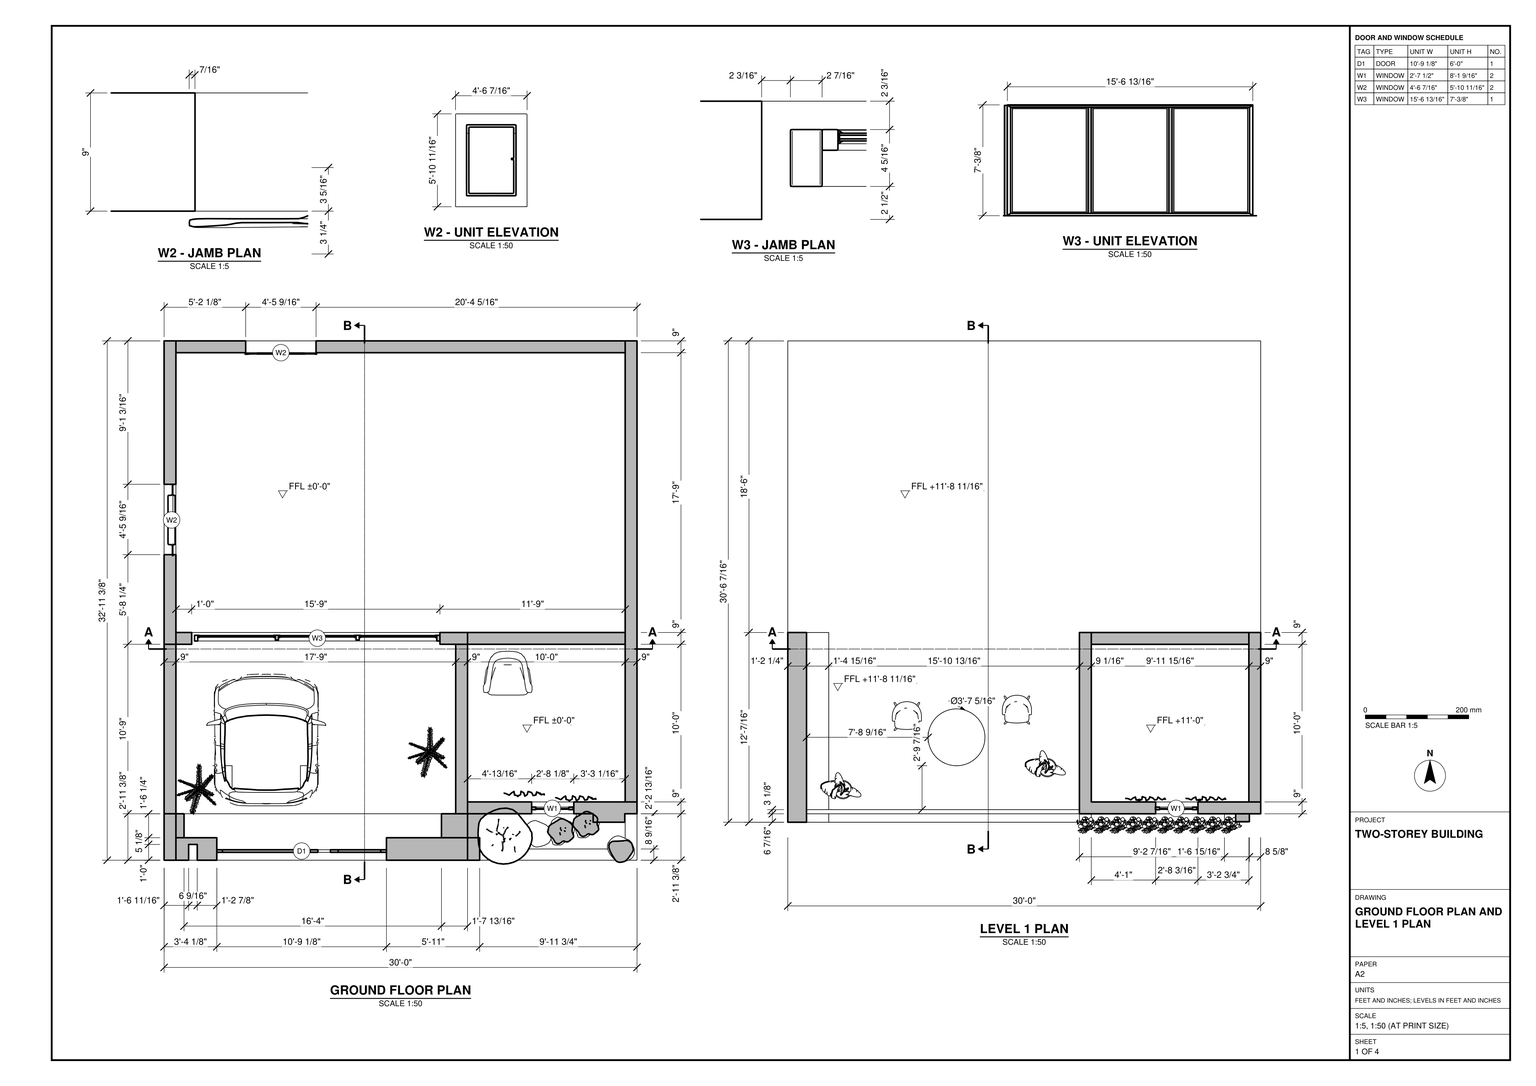
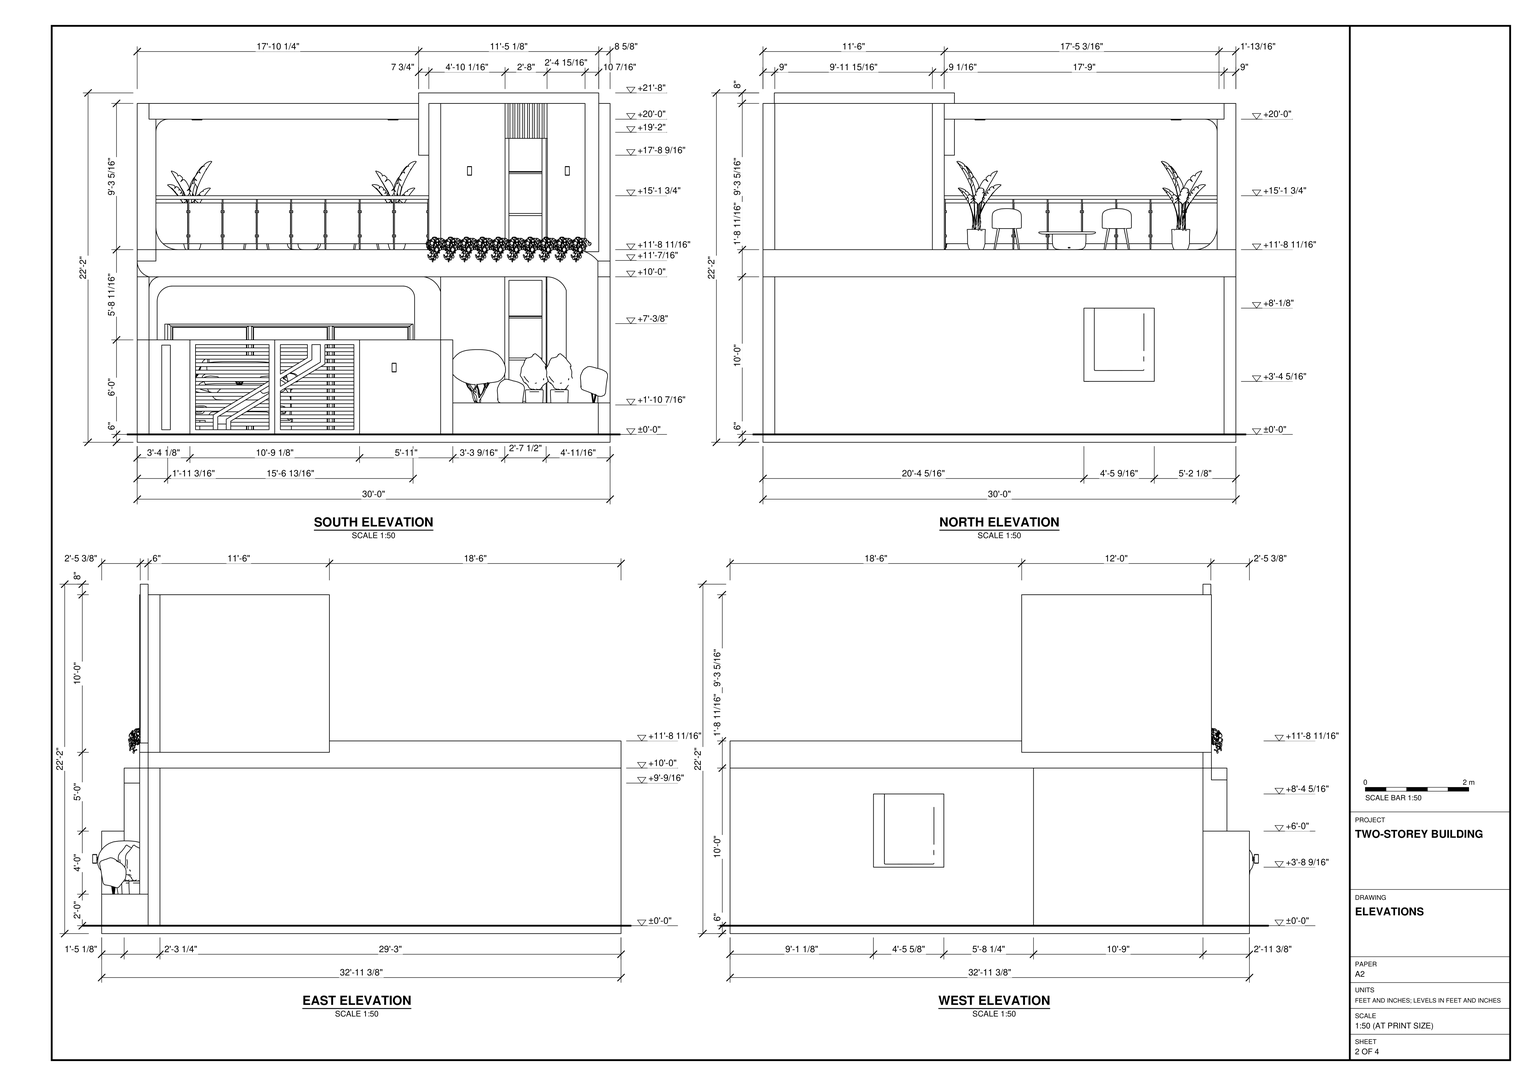
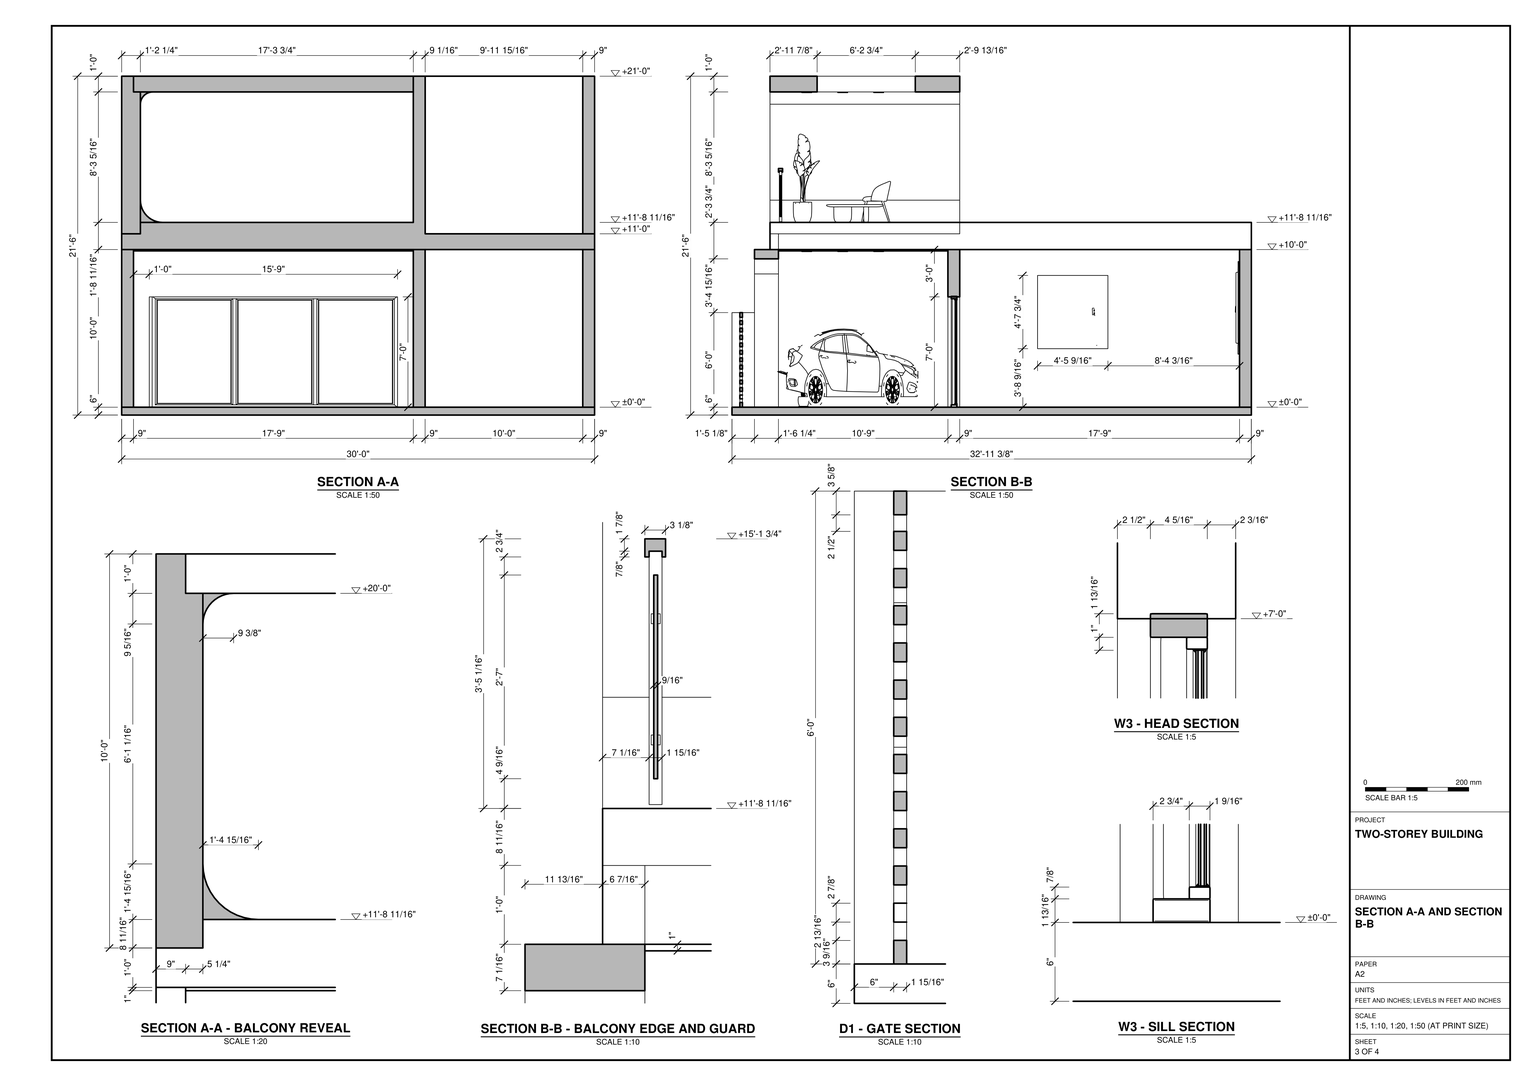
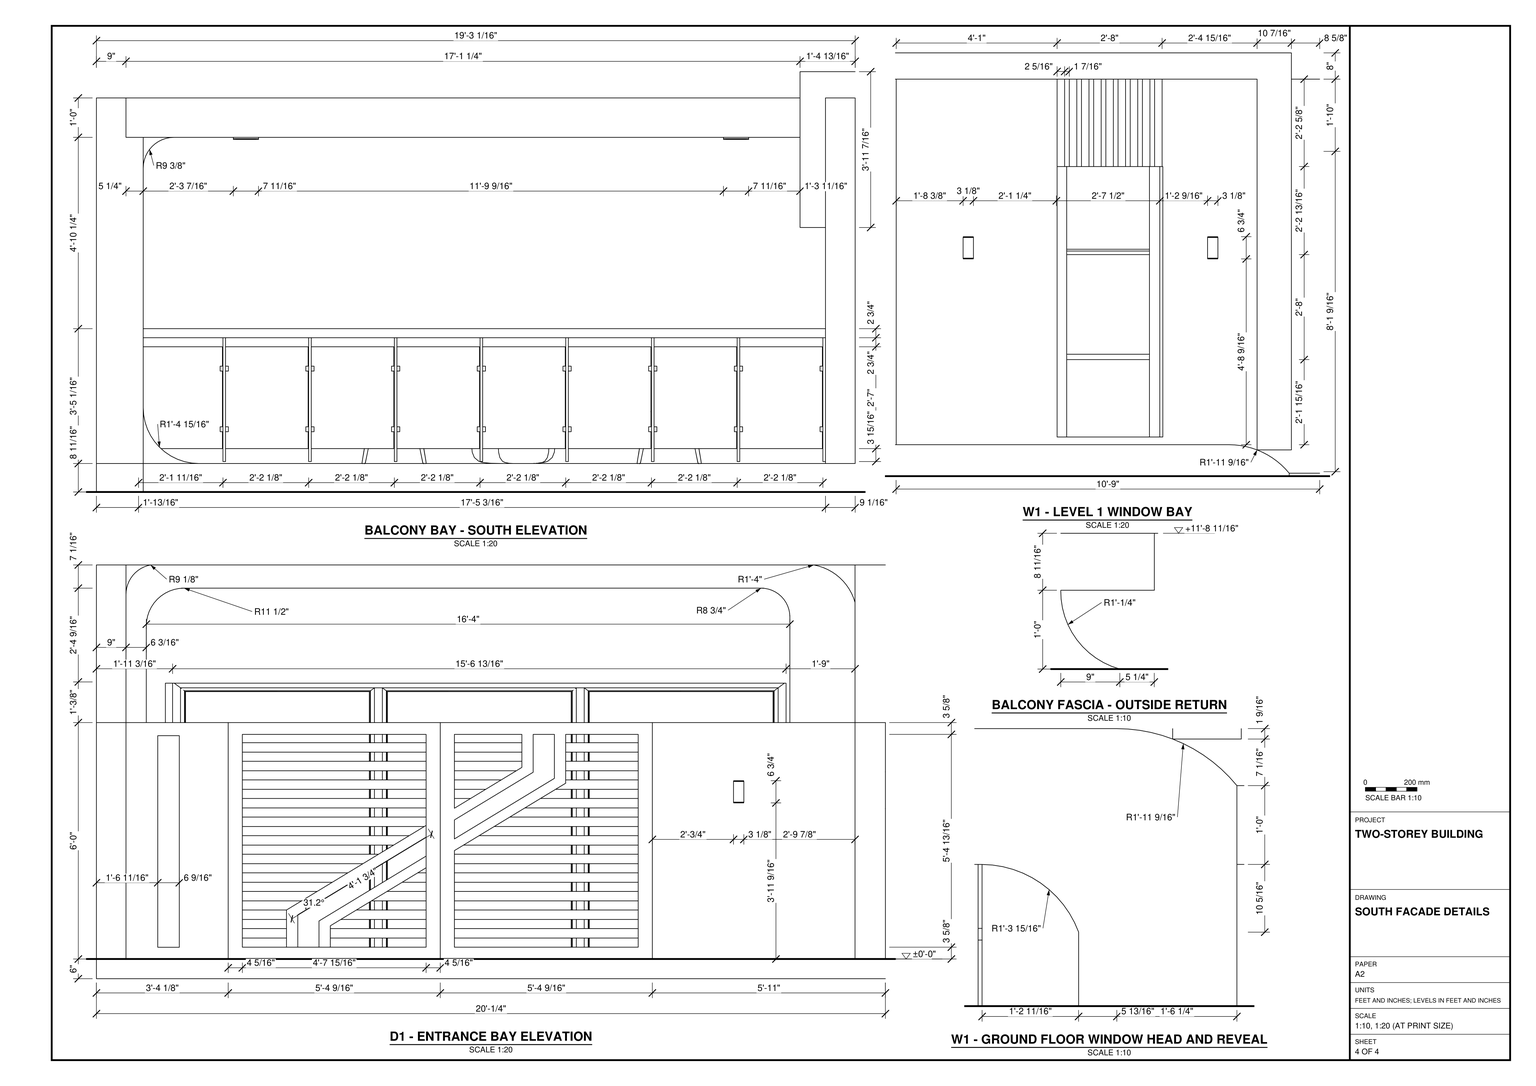
Build the two-storey building in SketchUp from task_files/diagram_01.pdf. Work in feet and inches. The overall model is 30'-0" wide, 33'-6 1/4" deep and 22'-2" high. Set the ground floor at ±0'-0" and the upper level at +11'-8 11/16".

Use the south elevation as the front. Lay out the large rear room, the covered parking bay at the front left and the smaller room at the front right. Model the walls at their drawn thicknesses, including the 9" walls shown in plan. Fit the slatted gate between the front wall piers and place the wide, three-panel window in the wall behind the parking bay. Use the plans and window schedule to locate and size the other window units.

Form the ground slab, upper slab and flat roof to match the sections. Keep the upper enclosure and covered balcony toward the front, leaving the roof surface visible behind them. Model the curved balcony reveals, stepped slab edge and glazed guard with its posts and top rail. Place the chairs and round table on the balcony, the car behind the gate and the planting as shown. Decor and loose items may be any suitable library component, for example from 3D Warehouse.

Keep the shell elements and each furniture or joinery piece in separate groups or components, and use components for repeated parts. Save one SketchUp model as output_files/two_storey_building_with_a_gated_carport_and_balcony.skp.

# SketchUp Ruby script. Lengths in inches.
U = 1.inch
M = Sketchup.active_model
def pt(a) = Geom::Point3d.new(a.map { |v| v * U })
def face(e, loops, mat)
  f = e.add_face(loops[0].map { |a| pt(a) })
  loops[1..].each { |l| e.add_face(l.map { |a| pt(a) }).erase! }
  f.material = f.back_material = mat if mat
  f
end
# faces: each face lists its corners as indices into pts; further lists are holes
def faces(e, pts, list, mat = nil) = list.each { |f| face(e, (f[0].is_a?(Array) ? f : [f]).map { |l| l.map { |i| pts[i] } }, mat) }
# xy, xz, yz: faces in a plane at the given z, y or x. An outline is a flat list of corners, or four numbers for a rectangle; further outlines are holes
def ring(l) = l.size == 4 ? [[l[0], l[1]], [l[2], l[1]], [l[2], l[3]], [l[0], l[3]]] : l.each_slice(2).to_a
def flat(e, list, mat, &to3) = list.each { |f| face(e, (f[0].is_a?(Array) ? f : [f]).map { |l| ring(l).map { |u, v| to3.(u, v) } }, mat) }
def xy(e, z, list, mat = nil) = flat(e, list, mat) { |x, y| [x, y, z] }
def xz(e, y, list, mat = nil) = flat(e, list, mat) { |x, z| [x, y, z] }
def yz(e, x, list, mat = nil) = flat(e, list, mat) { |y, z| [x, y, z] }
def lines(e, pts, list) = list.each { |a, b| e.add_line(pt(pts[a]), pt(pts[b])) }
# prism: a flat outline (further loops are holes) pulled along v
def prism(e, loops, v, mat = nil)
  f = face(e, loops, mat); d = Geom::Vector3d.new(v.map { |x| x * U })
  f.pushpull(f.normal.samedirection?(d) ? d.length : -d.length)
end
def box(e, o, s, mat = nil) = prism(e, [[o, [o[0] + s[0], o[1], o[2]], [o[0] + s[0], o[1] + s[1], o[2]], [o[0], o[1] + s[1], o[2]]]], [0, 0, s[2]], mat)
def at(x, y, z, deg = 0) = Geom::Transformation.translation(pt([x, y, z])) * Geom::Transformation.rotation(ORIGIN, Z_AXIS, deg.degrees)
def axes(o, x, y, z) = Geom::Transformation.new([*x, 0, *y, 0, *z, 0, *pt(o).to_a, 1])
def part(name) = M.definitions.add(name)
# library, detail: a bought-in or finely detailed component or shape, given as its bounding box
def library(name, o, s) = part(name).tap { |d| box(d.entities, o, s) }
def detail(e, o, s) = box(e.add_group.entities, o, s)
def put(e, d, t, mat = nil) = e.add_instance(d, t).tap { |i| i.material = mat if mat }
def group(e, t, mat = nil) = e.add_group.tap { |g| g.transformation = t; g.material = mat if mat }.entities
root = M.entities
M.materials.add("0210 AP 9427 DELICATE PINK").color = [242, 226, 232]
M.materials.add("Emissive").color = [221, 220, 187]
M.materials.add("Granite H 80cm").color = [113, 112, 109]
M.materials.add("Magma Rock Solid 19-98 100cm").color = [52, 53, 45]
M.materials.add("Marble Black 01 150cm").color = [31, 31, 31]
M.materials.add("[0131_Silver]").color = [28, 28, 28]
M.materials.add("[Translucent Glass Gray]").color = [128, 128, 128]
M.materials["[Translucent Glass Gray]"].alpha = 0.5
M.materials.add("[Translucent_Glass_Blue]").color = [255, 255, 255]
M.materials["[Translucent_Glass_Blue]"].alpha = 0
c1 = library("Window 109 011",[-27.22,-3.26,-0.09],[54.45,6.58,70.7])
c2 = library("Window 46-47",[-61.02,-2.17,0],[122.04,4.34,74.02])
c3 = library("Omni Light",[-12,-12,-12],[24,24,24])
c4 = library("Vavel Single Sofa",[-18.54,-16.85,0],[37.08,33.42,32.21])
c5 = part("Window")
xy(c5.entities,0,[[0,0,19.69,1.97]])
xy(c5.entities,1.97,[[1.97,0,17.72,0.79]])
xy(c5.entities,1.97,[[1.97,0.79,17.72,1.97]],"[Translucent Glass Gray]")
xy(c5.entities,24.8,[[1.97,0,17.72,0.79]])
xy(c5.entities,24.8,[[1.97,0.79,17.72,1.97]],"[Translucent Glass Gray]")
xy(c5.entities,25.98,[[1.97,0,17.72,0.79],[1.97,0.79,17.72,1.97]])
xy(c5.entities,48.03,[[1.97,0,17.72,1.97]])
xy(c5.entities,49.21,[[1.97,0,17.72,0.79]])
xy(c5.entities,49.21,[[1.97,0.79,17.72,1.97]],"[Translucent Glass Gray]")
xy(c5.entities,68.9,[[1.97,0,17.72,0.79]])
xy(c5.entities,68.9,[[1.97,0.79,17.72,1.97]],"[Translucent Glass Gray]")
xy(c5.entities,70.87,[[0,0,19.69,1.97]])
xz(c5.entities,0,[[[0,0,19.69,70.87],[1.97,1.97,17.72,68.9]]])
xz(c5.entities,0.79,[[1.97,1.97,17.72,24.8],[1.97,25.98,17.72,48.82],[1.97,49.21,17.72,68.9]],"[Translucent Glass Gray]")
xz(c5.entities,1.97,[[[0,0,19.69,70.87],[1.97,1.97,17.72,68.9]],[1.97,24.8,17.72,25.98],[1.97,48.03,17.72,49.21]])
yz(c5.entities,0,[[0,0,1.97,70.87]])
yz(c5.entities,1.97,[[0,1.97,0.79,24.8],[0,24.8,1.97,25.98],[0,25.98,0.79,48.03],[0.79,25.98,1.97,48.03],[0,48.03,1.97,49.21],
  [0,49.21,0.79,68.9]])
yz(c5.entities,1.97,[[0.79,1.97,1.97,24.8],[0.79,49.21,1.97,68.9]],"[Translucent Glass Gray]")
yz(c5.entities,17.72,[[0,1.97,0.79,24.8],[0,24.8,1.97,25.98],[0,25.98,0.79,48.03],[0.79,25.98,1.97,48.03],[0,48.03,1.97,49.21],
  [0,49.21,0.79,68.9]])
yz(c5.entities,17.72,[[0.79,1.97,1.97,24.8],[0.79,49.21,1.97,68.9]],"[Translucent Glass Gray]")
yz(c5.entities,19.69,[[0,0,1.97,70.87]])
c6 = library("Curtains 004",[-15.59,-2.26,0],[31.18,4.52,116.91])
c7 = library("Omni Light\#1",[-12,-12,-12],[24,24,24])
c8 = library("Modern Gate 1",[0,0,0],[118.11,1.97,78.74])
c9 = library("2016+Honda+Civic+LX+Sedan",[0.01,0.03,0.02],[16.17,34.46,10.62])
c10 = library("Tsuki Coffee Table",[-21.63,-21.63,0],[43.26,43.26,13.58])
c11 = library("Chair 293 011 002",[-11.125,-11.03,-0.12],[22.25,22.06,31.4])
c12 = library("Plant 260 020",[-18.86,-7.03,0.01],[33.61,20.04,67.26])
c13 = library("Potted Plant 02",[-16.98,-19.78,0],[30.04,38.68,37.52])
c14 = library("Peperomia 450 001",[-6.6875,-10.1875,-9.42],[16.7,12.74,19.03])
c15 = library("Wall Light 02",[0,0,0],[3.15,6.76,4.53])
c16 = library("Spot Light",[-5.1,-5.1,-11.05],[10.2,10.2,11.05])
c17 = library("Juniperus sabina Monna 005",[-21.09,-21.39,-0.1875],[42.47,43.11,50.49])
c18 = library("Cyperus alternifolius 005",[-10.04,-10.17,-0.01],[20.71,20.19,27.77])
c19 = library("Potted Plant 60-25",[-10.7,-10.47,0],[21.2,21.27,47.12])
c20 = part("Group\#2")
xy(c20.entities,0,[[0,0,0.39,2.125]],"[0131_Silver]")
xy(c20.entities,1.5,[[0,0,0.39,2.125]],"[0131_Silver]")
xz(c20.entities,0,[[0,0,0.39,1.5]],"[0131_Silver]")
xz(c20.entities,2.125,[[0,0,0.39,1.5]],"[0131_Silver]")
yz(c20.entities,0,[[0,0,2.125,1.5]],"[0131_Silver]")
yz(c20.entities,0.39,[[0,0,2.125,1.5]],"[0131_Silver]")
c21 = part("Glass railing panel")
xy(c21.entities,0,[[-0.59,0,0,63.98]])
xy(c21.entities,37.71,[[-0.59,0,0,63.98]])
xz(c21.entities,0,[[-0.59,0,0,37.71]])
xz(c21.entities,63.98,[[-0.59,0,0,37.71]])
yz(c21.entities,-0.59,[[0,0,63.98,37.71]])
yz(c21.entities,0,[[0,0,63.98,0,63.98,37.71,0,37.71,0,30.53,1.75,30.53,1.75,28.71,0,28.71],[-0.4,28.71,0,30.53],[0,28.71,1.75,30.53]])
p = [[0,63.98,30.53],[0.39,63.98,30.53]]
lines(c21.entities,p,[[0,1]])
put(c21.entities,c20,axes([0,62.22,28.71],[1,0,0],[0,1.01246,0],[0,0,1.2158]))
put(c21.entities,c20,axes([0,62.22,6.27],[1,0,0],[0,1.01246,0],[0,0,1.2158]))
put(c21.entities,c20,axes([0,0.6,28.71],[1,0,0],[0,1.01246,0],[0,0,1.2158]))
put(c21.entities,c20,axes([0,0.6,6.27],[1,0,0],[0,1.01246,0],[0,0,1.2158]))
put(c21.entities,c20,axes([-0.98,0.6,28.71],[1,0,0],[0,1.01246,0],[0,0,1.2158]))
put(c21.entities,c20,axes([-0.98,62.22,6.27],[1,0,0],[0,1.01246,0],[0,0,1.2158]))
put(c21.entities,c20,axes([-0.98,0.6,6.27],[1,0,0],[0,1.01246,0],[0,0,1.2158]))
put(c21.entities,c20,axes([-0.98,62.22,28.71],[1,0,0],[0,1.01246,0],[0,0,1.2158]))
c22 = part("Group\#3")
xz(c22.entities,0,[[0,0,1.97,38.58]])
xz(c22.entities,1.97,[[0,0,1.97,38.58]])
yz(c22.entities,0,[[0,0,1.97,37.71]])
yz(c22.entities,1.97,[[0,0,1.97,37.71]])
c23 = part("Glass balcony railing")
xy(c23.entities,37.71,[[2.51,0,3.15,0.39,3.15,0]])
xy(c23.entities,37.71,[[0,0,0.54,520.67],[2.51,0,2.51,63.58,3.15,0.39],[3.15,0.39,2.51,63.58,2.51,520.67,3.15,520.67]],"[0131_Silver]")
xy(c23.entities,38.58,[[0.54,496.0625,2.51,520.67]])
xy(c23.entities,38.58,[[0.54,0,2.51,496.0625]],"[0131_Silver]")
xy(c23.entities,40.46,[[0,0,3.15,520.67]],"[0131_Silver]")
xz(c23.entities,0,[[0,37.71,0.54,37.71,0.54,38.58,2.51,38.58,2.51,37.71,3.15,37.71,3.15,40.46,0,40.46]],"[0131_Silver]")
xz(c23.entities,520.67,[[0,37.71,0,40.46,3.15,40.46,3.15,37.71,2.51,37.71,2.51,38.58,0.54,38.58,0.54,37.71]])
yz(c23.entities,0,[[0,37.71,520.67,40.46]],"[0131_Silver]")
yz(c23.entities,0.54,[[496.0625,37.71,520.67,38.58]])
yz(c23.entities,0.54,[[0,37.71,496.0625,38.58]],"[0131_Silver]")
yz(c23.entities,2.51,[[0,37.71,496.0625,38.58],[496.0625,37.71,520.67,38.58]])
yz(c23.entities,3.15,[[0,37.71,520.67,40.46]],"[0131_Silver]")
put(c23.entities,c21,axes([1.8,65.35,3.9375],[1,0,0],[0,0.98769,0],[0,0,0.8225]),"[Translucent_Glass_Blue]")
put(c23.entities,c21,axes([1.8,130.31,3.9375],[1,0,0],[0,0.98769,0],[0,0,0.8225]),"[Translucent_Glass_Blue]")
put(c23.entities,c21,axes([1.8,195.28,3.9375],[1,0,0],[0,0.98769,0],[0,0,0.8225]),"[Translucent_Glass_Blue]")
put(c23.entities,c21,axes([1.8,260.24,3.9375],[1,0,0],[0,0.98769,0],[0,0,0.8225]),"[Translucent_Glass_Blue]")
put(c23.entities,c21,axes([1.8,325.2,3.9375],[1,0,0],[0,0.98769,0],[0,0,0.8225]),"[Translucent_Glass_Blue]")
put(c23.entities,c21,axes([1.8,390.16,3.9375],[1,0,0],[0,0.98769,0],[0,0,0.8225]),"[Translucent_Glass_Blue]")
put(c23.entities,c21,axes([1.8,455.12,3.9375],[1,0,0],[0,0.98769,0],[0,0,0.8225]),"[Translucent_Glass_Blue]")
put(c23.entities,c21,axes([1.8,0.39,3.9375],[1,0,0],[0,0.98769,0],[0,0,0.8225]),"[Translucent_Glass_Blue]")
put(c23.entities,c22,at(0.54,128.9375,0),"[0131_Silver]")
g1 = group(c23.entities,at(0.54,63.98,0),"[0131_Silver]")
xz(g1,0,[[0,0,1.97,38.58]])
xz(g1,1.97,[[0,0,1.97,38.58]])
yz(g1,0,[[0,0,1.97,37.71]])
yz(g1,1.97,[[0,0,1.97,37.71]])
put(c23.entities,c22,at(0.54,193.9,0),"[0131_Silver]")
put(c23.entities,c22,at(0.54,258.86,0),"[0131_Silver]")
put(c23.entities,c22,at(0.54,323.82,0),"[0131_Silver]")
put(c23.entities,c22,at(0.54,388.78,0),"[0131_Silver]")
put(c23.entities,c22,at(0.54,453.74,0),"[0131_Silver]")
put(c23.entities,c22,at(0.54,518.7,0),"[0131_Silver]")
c24 = part("Glass+Railing")
put(c24.entities,c23,axes([0,0,0],[1,0,0],[0,0.95652,0],[0,0,1]),"[0131_Silver]")
c25 = library("Tlon Light 650 Ceiling 152 007",[-12.8,-12.8,-3.78],[25.6,25.6,3.58])
xy(root,-6,[[0,0,360,395.375]])
xy(root,0,[[0,0,9,35.375],[9,0,40.125,17.125],[169.28,0,231,17.125],[231,0,240.25,17.125],[240.25,0,351,8.5625],
  [351,0,360,35.375],[9,17.125,15.1875,35.375],[211.16,17.125,231,35.375],[326.61,28.9375,350.71,28.9375,350.71,35.375,351,35.375,351,44.375,231,44.375,231,35.375,326.61,35.375],[0,35.375,9,164.375],
  [9,35.375,222,35.375,222,164.375,210,164.375,210,173.375,21,173.375,21,164.375,9,164.375],[222,35.375,231,164.375],[351,35.375,360,44.375],[231,44.375,351,164.375],[351,44.375,360,395.375],
  [0,164.375,9,395.375],[9,164.375,21,173.375],[210,164.375,231,173.375],[210,164.375,231,173.375],[231,164.375,351,173.375],
  [9,173.375,351,386.375],[9,386.375,351,395.375]])
xy(root,0,[[40.125,0,169.28,0,169.28,17.125,211.16,17.125,211.16,35.375,15.1875,35.375,15.1875,17.125,40.125,17.125]],"Granite H 80cm")
xy(root,3.57,[[18.68,0,25.24,12]],"Emissive")
xy(root,14.3125,[[240.25,8.5625,351,8.5625,351,35.375,350.71,35.375,350.71,28.9375,326.61,28.9375,326.61,35.375,231,35.375,231,17.125,240.25,17.125]],"Granite H 80cm")
xy(root,22.46,[[279.81,35.375,311.91,44.375]])
xy(root,24,[[240.25,0,351,8.5625],[351,0,360,35.375]],"Granite H 80cm")
xy(root,40.39,[[62.12,386.375,115.68,395.375]])
xy(root,44.55,[[0,232.62,9,286.18]])
xy(root,68.01,[[18.68,0,25.24,12]],"Emissive")
xy(root,72,[[169.28,0,231,17.125],[231,0,240.25,17.125]],"Granite H 80cm")
xy(root,72,[[0,0,9,35.375],[9,0,40.125,17.125]],"Marble Black 01 150cm")
xy(root,84,[[21,164.375,210,173.375]])
xy(root,96.14,[[62.12,386.375,115.68,395.375]])
xy(root,100.3,[[0,232.62,9,286.18]])
xy(root,112.9375,[[26.67,17.125,202.38,35.375]],"Marble Black 01 150cm")
xy(root,119,[[9,35.375,222,164.375]],"0210 AP 9427 DELICATE PINK")
xy(root,120,[[9,28.9375,231,35.375],[231,28.9375,279.81,35.375],[279.81,28.9375,279.81,44.375,231,44.375,231,164.375,351,164.375,351,44.375,311.91,44.375,311.91,28.9375],[0,35.375,9,164.375],[9,35.375,222,164.375],
  [222,35.375,231,164.375],[231,35.375,279.81,44.375],[351,35.375,360,44.375],[351,44.375,360,395.375],[0,164.375,9,395.375],
  [9,164.375,231,173.375],[231,164.375,351,173.375],[9,173.375,351,386.375],[9,386.375,351,395.375]])
xy(root,120,[[16.46,17.125,218.45,28.9375]],"Marble Black 01 150cm")
xy(root,132,[[0,28.9375,14.25,173.375],[231.04,44.375,351,164.375],[351,44.375,360,173.375],[231.04,164.375,351,173.375]])
xy(root,139.09,[[340.93,29.375,351.375,35.375]])
xy(root,140.68,[[31.18,28.9375,222,28.9375,222,173.375,360,173.375,360,395.375,0,395.375,0,173.375,31.18,173.375],[14.25,28.9375,31.18,173.375],[222,28.9375,231.04,35.375],[231.04,28.9375,332.43,35.375]])
xy(root,143.02,[[280.04,35.375,312.22,44.375]])
xy(root,212.55,[[214.26,29.375,222,35.375]])
xy(root,225.38,[[280.04,35.375,312.22,44.375]])
xy(root,240,[[9,28.9375,14.25,173.375],[14.25,28.9375,23.6,173.375]])
xy(root,240,[[[23.6,28.9375,23.6,173.375,222,173.375,222,35.375,214.26,35.375,214.26,28.9375],[123.04,54.3,135.4375,55.86,147.01,60.58,156.97,68.13,164.64,78,169.49,89.52,171.1875,101.9,169.63,114.3,164.91,125.875,157.36,135.84,147.49,143.5,135.97,148.35,123.59,150.05,111.19,148.49,99.62,143.78,89.66,136.23,81.99,126.36,77.14,114.84,75.44,102.46,77,90.06,81.72,78.48,89.27,68.52,99.14,60.86,110.66,56.01]]],"0210 AP 9427 DELICATE PINK")
xy(root,252,[[0,28.9375,9,173.375],[[9,28.9375,214.26,28.9375,214.26,35.375,222,35.375,222,173.375,9,173.375],[123.04,54.3,110.66,56.01,99.14,60.86,89.27,68.52,81.72,78.48,77,90.06,75.44,102.46,77.14,114.84,81.99,126.36,89.66,136.23,99.62,143.78,111.19,148.49,123.59,150.05,135.97,148.35,147.49,143.5,157.36,135.84,164.91,125.875,169.63,114.3,171.1875,101.9,169.49,89.52,164.64,78,156.97,68.13,147.01,60.58,135.4375,55.86]],[231.04,164.375,351,173.375]])
xy(root,252,[[222,35.375,231.04,173.375],[231.04,35.375,360,44.375],[231.04,44.375,351,164.375],[351,44.375,360,173.375]],"Granite H 80cm")
xy(root,252,[[222,29.375,340.93,35.375]],"Magma Rock Solid 19-98 100cm")
xy(root,260,[[214.26,29.375,351.375,35.375]])
xz(root,0,[[0,-6,360,0],[169.28,0,231,72],[231,0,240.25,72],[240.25,0,351,24],[351,0,360,24]],"Granite H 80cm")
xz(root,0,[[0,0,9,72],[[9,0,40.125,72],[18.68,3.57,25.24,68.01]]],"Marble Black 01 150cm")
xz(root,8.5625,[[240.25,0,351,14.3125],[240.25,14.3125,351,24]])
xz(root,12,[[18.68,3.57,25.24,68.01]],"Emissive")
xz(root,17.125,[[9,0,15.1875,72],[15.1875,0,40.125,72],[169.28,0,211.16,72],[211.16,0,231,72],[231,0,240.25,14.3125],
  [231,14.3125,240.25,72]])
xz(root,17.125,[[9,72,15.1875,72,15.1875,101.45,15.29,102.95,15.58,104.43,16.0625,105.85,16.73,107.19,17.56,108.44,18.55,109.57,19.68,110.5625,20.93,111.4,22.28,112.0625,23.7,112.55,25.17,112.84,26.67,112.9375,202.38,112.9375,203.53,112.86,204.65,112.64,205.74,112.27,206.77,111.76,207.72,111.12,208.59,110.37,209.34,109.5,209.98,108.55,210.49,107.52,210.86,106.43,211.08,105.31,211.16,104.16,211.16,72,231,72,231,108.58,230.53,110,229.93,111.36,229.21,112.67,228.37,113.9,227.42,115.04,226.36,116.1,225.21,117.05,223.98,117.89,222.68,118.61,221.3125,119.2,219.9,119.67,218.45,120,16.46,120,15.4375,119.75,14.45,119.375,13.51,118.89,12.63,118.31,11.83,117.62,11.11,116.85,10.48,116,9.96,115.08,9.54,114.11,9.24,113.1,9.0625,112.0625,9,111.01]],"Marble Black 01 150cm")
xz(root,28.9375,[[326.61,0,350.71,14.3125],[0,132,14.25,140.68],[14.25,140.68,31.18,140.68,28.97,140.82,26.8,141.25,24.7,141.97,22.72,142.95,20.875,144.18,19.21,145.64,17.75,147.3,16.52,149.14,15.54,151.13,14.83,153.23,14.39,155.4,14.25,157.61]])
xz(root,28.9375,[[326.61,14.3125,350.71,14.3125,350.71,132,349.56,133.31,348.31,134.53,346.98,135.65,345.57,136.68,344.09,137.59,342.55,138.4,340.95,139.09,339.3,139.65,337.62,140.1,335.9,140.42,334.17,140.61,332.43,140.68,14.25,140.68,14.25,132,0,132,0.05,130.66,0.25,129.33,0.6,128.03,1.08,126.77,1.7,125.58,2.45,124.46,3.3125,123.43,4.29,122.5,5.35,121.6875,6.51,120.99,7.73,120.43,9,120,311.91,120,313.5,119.91,315.07,119.66,316.61,119.25,318.1,118.69,319.52,117.98,320.87,117.14,322.125,116.16,323.27,115.0625,324.31,113.85,325.22,112.55,325.99,111.15,326.61,109.69],[0,140.68,14.25,140.68,14.25,240,9,240,9,252,0,252],[14.25,230.65,14.33,231.875,14.57,233.07,14.96,234.23,15.5,235.33,16.18,236.34,16.99,237.26,17.91,238.07,18.92,238.75,20.02,239.29,21.18,239.68,22.375,239.92,23.6,240,14.25,240],[9,240,214.26,252]],"0210 AP 9427 DELICATE PINK")
xz(root,28.9375,[[231,108.58,231,120,218.45,120,219.9,119.67,221.3125,119.2,222.68,118.61,223.98,117.89,225.21,117.05,226.36,116.1,227.42,115.04,228.37,113.9,229.21,112.67,229.93,111.36,230.53,110],[9,111.01,9.0625,112.0625,9.24,113.1,9.54,114.11,9.96,115.08,10.48,116,11.11,116.85,11.83,117.62,12.63,118.31,13.51,118.89,14.45,119.375,15.4375,119.75,16.46,120,9,120]],"Marble Black 01 150cm")
xz(root,29.375,[[340.93,139.09,351.375,139.09,351.375,260,214.26,260,214.26,212.55,222,212.55,222,252,340.93,252]],"Magma Rock Solid 19-98 100cm")
xz(root,35.375,[[0,0,9,72],[9,0,9,119,222,119,222,0,211.16,0,211.16,112.9375,15.1875,112.9375,15.1875,0],[222,0,231,119],[231,0,326.61,14.3125],[350.71,0,351,14.3125],
  [351,0,360,24],[15.1875,101.45,15.1875,112.9375,26.67,112.9375,25.17,112.84,23.7,112.55,22.28,112.0625,20.93,111.4,19.68,110.5625,18.55,109.57,17.56,108.44,16.73,107.19,16.0625,105.85,15.58,104.43,15.29,102.95],[211.16,104.16,211.08,105.31,210.86,106.43,210.49,107.52,209.98,108.55,209.34,109.5,208.59,110.37,207.72,111.12,206.77,111.76,205.74,112.27,204.65,112.64,203.53,112.86,202.38,112.9375,211.16,112.9375],[9,119,222,120],[222,119,231,120],
  [340.93,139.09,351.375,252],[214.26,212.55,222,240],[280.04,225.38,282.32,252],[282.32,225.38,283.75,252],[283.75,225.38,286.03,252],
  [286.03,225.38,287.46,252],[287.46,225.38,289.74,252],[289.74,225.38,291.17,252],[291.17,225.38,293.46,252],[293.46,225.38,294.88,252],
  [294.88,225.38,297.17,252],[297.17,225.38,298.59,252],[298.59,225.38,300.875,252],[300.875,225.38,302.3,252],[302.3,225.38,304.59,252],
  [304.59,225.38,306.01,252],[306.01,225.38,308.3,252],[308.3,225.38,309.72,252],[309.72,225.38,312.01,252],[214.26,240,222,252],
  [214.26,252,351.375,260]])
xz(root,35.375,[[0,72,9,120],[0,120,9,120,7.73,120.43,6.51,120.99,5.35,121.6875,4.29,122.5,3.3125,123.43,2.45,124.46,1.7,125.58,1.08,126.77,0.6,128.03,0.25,129.33,0.05,130.66,0,132]],"0210 AP 9427 DELICATE PINK")
xz(root,35.375,[[350.71,14.3125,351,14.3125,351,24,360,24,360,120,350.71,120],[350.71,120,360,132],[350.71,132,360,132,360,252,351.375,252,351.375,139.09,340.93,139.09,340.95,139.09,342.55,138.4,344.09,137.59,345.57,136.68,346.98,135.65,348.31,134.53,349.56,133.31]],"Granite H 80cm")
xz(root,35.375,[[231,14.3125,326.61,14.3125,326.61,109.69,325.99,111.15,325.22,112.55,324.31,113.85,323.27,115.0625,322.125,116.16,320.87,117.14,319.52,117.98,318.1,118.69,316.61,119.25,315.07,119.66,313.5,119.91,311.91,120,311.91,22.46,279.81,22.46,279.81,120,231,120],[340.93,139.09,340.93,252,312.01,252,312.01,225.38,312.22,225.38,312.22,143.02,280.04,143.02,280.04,252,231.04,252,231.04,140.68,332.43,140.68,334.17,140.61,335.9,140.42,337.62,140.1,339.3,139.65],[222,140.68,231.04,252]],"Marble Black 01 150cm")
xz(root,44.375,[[231,0,231,120,279.81,120,279.81,22.46,311.91,22.46,311.91,120,351,120,351,0],[351,0,360,120],[[231.04,132,351,252],[280.04,143.02,312.22,225.38]],[351,132,360,252]])
xz(root,164.375,[[0,0,9,120],[222,0,231,120],[231,0,351,120],[9,119,222,120],[231.04,132,351,252]])
xz(root,164.375,[[9,0,21,0,21,84,210,84,210,0,222,0,222,119,9,119]],"0210 AP 9427 DELICATE PINK")
xz(root,173.375,[[9,0,9,120,231,120,231,0,210,0,210,84,21,84,21,0],[231,0,351,120],[0,132,14.25,140.68],[222,132,231.04,140.68],[231.04,132,351,140.68],
  [351,132,360,140.68],[0,140.68,0,252,9,252,9,240,14.25,240,14.25,140.68],[14.25,140.68,14.25,157.61,14.39,155.4,14.83,153.23,15.54,151.13,16.52,149.14,17.75,147.3,19.21,145.64,20.875,144.18,22.72,142.95,24.7,141.97,26.8,141.25,28.97,140.82,31.18,140.68],[222,140.68,231.04,252],[231.04,140.68,351,252],
  [351,140.68,360,252],[14.25,230.65,14.25,240,23.6,240,22.375,239.92,21.18,239.68,20.02,239.29,18.92,238.75,17.91,238.07,16.99,237.26,16.18,236.34,15.5,235.33,14.96,234.23,14.57,233.07,14.33,231.875],[9,240,222,252]])
xz(root,232.62,[[0,44.55,9,100.3]])
xz(root,286.18,[[0,44.55,9,100.3]])
xz(root,386.375,[[[9,0,351,120],[62.12,40.39,115.68,96.14]]])
xz(root,395.375,[[0,-6,360,0],[0,0,9,120],[[9,0,351,120],[62.12,40.39,115.68,96.14]],[351,0,360,120],[0,120,360,140.68]])
yz(root,0,[[0,-6,395.375,0],[35.375,0,164.375,120],[[164.375,0,395.375,120],[232.62,44.55,286.18,100.3]],[35.375,120,35.375,132,173.375,132,173.375,140.68,395.375,140.68,395.375,120],[28.9375,132,173.375,252]])
yz(root,0,[[0,0,35.375,72]],"Marble Black 01 150cm")
yz(root,9,[[0,0,17.125,72],[17.125,0,35.375,72],[164.375,0,173.375,120],[[173.375,0,386.375,120],[232.62,44.55,286.18,100.3]],[386.375,0,395.375,120],
  [35.375,119,164.375,120],[28.9375,240,173.375,252]])
yz(root,9,[[35.375,0,164.375,119]],"0210 AP 9427 DELICATE PINK")
yz(root,9,[[17.125,72,17.125,111.01,28.9375,111.01,28.9375,120,35.375,120,35.375,72]],"Marble Black 01 150cm")
yz(root,14.25,[[28.9375,132,173.375,140.68],[28.9375,140.68,173.375,157.61],[28.9375,230.65,173.375,240]])
yz(root,14.25,[[28.9375,157.61,173.375,230.65]],"0210 AP 9427 DELICATE PINK")
yz(root,15.1875,[[17.125,0,35.375,101.45]],"Marble Black 01 150cm")
yz(root,18.68,[[0,3.57,12,68.01]],"Emissive")
yz(root,21,[[164.375,0,173.375,84]])
yz(root,25.24,[[0,3.57,12,68.01]],"Emissive")
yz(root,40.125,[[0,0,17.125,72]],"0210 AP 9427 DELICATE PINK")
yz(root,62.12,[[386.375,40.39,395.375,96.14]])
yz(root,115.68,[[386.375,40.39,395.375,96.14]])
yz(root,169.28,[[0,0,17.125,72]])
yz(root,210,[[164.375,0,173.375,84]])
yz(root,211.16,[[17.125,0,35.375,104.16]],"Marble Black 01 150cm")
yz(root,214.26,[[28.9375,240,29.375,252],[29.375,240,35.375,252]])
yz(root,214.26,[[29.375,212.55,35.375,240],[29.375,252,35.375,260]],"Magma Rock Solid 19-98 100cm")
yz(root,222,[[35.375,119,164.375,120],[35.375,140.68,173.375,240],[29.375,212.55,35.375,252],[35.375,240,173.375,252]])
yz(root,222,[[35.375,0,164.375,119]],"0210 AP 9427 DELICATE PINK")
yz(root,231,[[0,0,17.125,72],[17.125,0,35.375,14.3125],[35.375,0,44.375,120],[44.375,0,164.375,120],[164.375,0,173.375,120]])
yz(root,231,[[17.125,14.3125,35.375,14.3125,35.375,120,28.9375,120,28.9375,108.58,17.125,108.58]],"0210 AP 9427 DELICATE PINK")
yz(root,231.04,[[44.375,132,164.375,252],[164.375,132,173.375,252]])
yz(root,240.25,[[0,0,8.5625,24],[8.5625,0,17.125,14.3125]])
yz(root,240.25,[[8.5625,14.3125,17.125,14.3125,17.125,72,0,72,0,24,8.5625,24]],"0210 AP 9427 DELICATE PINK")
yz(root,279.81,[[35.375,22.46,44.375,120]])
yz(root,280.04,[[35.375,143.02,44.375,225.38]])
yz(root,311.91,[[35.375,22.46,44.375,120]])
yz(root,312.22,[[35.375,143.02,44.375,225.38]])
yz(root,326.61,[[28.9375,0,35.375,14.3125],[28.9375,14.3125,35.375,109.69]])
yz(root,340.93,[[29.375,139.09,35.375,252]],"Magma Rock Solid 19-98 100cm")
yz(root,350.71,[[28.9375,0,35.375,14.3125],[28.9375,14.3125,35.375,120],[28.9375,120,35.375,132]])
yz(root,351,[[0,0,8.5625,24],[8.5625,0,35.375,14.3125],[44.375,0,164.375,120],[164.375,0,173.375,120],[173.375,0,386.375,120],
  [386.375,0,395.375,120],[8.5625,14.3125,35.375,24],[44.375,132,164.375,252],[164.375,132,173.375,252]])
yz(root,351.375,[[29.375,139.09,35.375,260]],"Magma Rock Solid 19-98 100cm")
yz(root,360,[[0,-6,395.375,0],[0,0,35.375,24]])
yz(root,360,[[35.375,0,44.375,120],[44.375,0,395.375,120],[35.375,120,395.375,120,395.375,140.68,173.375,140.68,173.375,132,35.375,132],[35.375,132,44.375,252],[44.375,132,173.375,252]],"Granite H 80cm")
p = [[15.29,17.125,102.95],[15.1875,17.125,101.45],[15.1875,35.375,101.45],[15.29,35.375,102.95],[15.58,17.125,104.43],[15.58,35.375,104.43],
  [211.16,17.125,104.16],[211.08,17.125,105.31],[211.08,35.375,105.31],[211.16,35.375,104.16],[16.0625,17.125,105.85],[16.0625,35.375,105.85],
  [210.86,17.125,106.43],[210.86,35.375,106.43],[16.73,17.125,107.19],[16.73,35.375,107.19],[210.49,17.125,107.52],[210.49,35.375,107.52],
  [17.56,17.125,108.44],[17.56,35.375,108.44],[209.98,17.125,108.55],[209.98,35.375,108.55],[18.55,17.125,109.57],[18.55,35.375,109.57],
  [209.34,17.125,109.5],[209.34,35.375,109.5],[230.53,17.125,110],[231,17.125,108.58],[231,28.9375,108.58],[230.53,28.9375,110],
  [208.59,17.125,110.37],[208.59,35.375,110.37],[19.68,17.125,110.5625],[19.68,35.375,110.5625],[325.99,35.375,111.15],[326.61,35.375,109.69],
  [326.61,28.9375,109.69],[325.99,28.9375,111.15],[229.93,17.125,111.36],[229.93,28.9375,111.36],[207.72,17.125,111.12],[207.72,35.375,111.12],
  [20.93,17.125,111.4],[20.93,35.375,111.4],[9,17.125,111.01],[9.0625,17.125,112.0625],[9.0625,28.9375,112.0625],[9,28.9375,111.01],
  [206.77,17.125,111.76],[206.77,35.375,111.76],[325.22,35.375,112.55],[325.22,28.9375,112.55],[22.28,17.125,112.0625],[22.28,35.375,112.0625],
  [229.21,17.125,112.67],[229.21,28.9375,112.67],[205.74,17.125,112.27],[205.74,35.375,112.27],[9.24,17.125,113.1],[9.24,28.9375,113.1],
  [23.7,17.125,112.55],[23.7,35.375,112.55],[204.65,17.125,112.64],[204.65,35.375,112.64],[25.17,17.125,112.84],[25.17,35.375,112.84],
  [324.31,35.375,113.85],[324.31,28.9375,113.85],[203.53,17.125,112.86],[203.53,35.375,112.86],[228.37,17.125,113.9],[228.37,28.9375,113.9],
  [26.67,17.125,112.9375],[26.67,35.375,112.9375],[202.38,17.125,112.9375],[202.38,35.375,112.9375],[9.54,17.125,114.11],[9.54,28.9375,114.11],
  [227.42,17.125,115.04],[227.42,28.9375,115.04],[323.27,35.375,115.0625],[323.27,28.9375,115.0625],[9.96,17.125,115.08],[9.96,28.9375,115.08],
  [226.36,17.125,116.1],[226.36,28.9375,116.1],[10.48,17.125,116],[10.48,28.9375,116],[322.125,35.375,116.16],[322.125,28.9375,116.16],
  [11.11,17.125,116.85],[11.11,28.9375,116.85],[225.21,17.125,117.05],[225.21,28.9375,117.05],[320.87,35.375,117.14],[320.87,28.9375,117.14],
  [11.83,17.125,117.62],[11.83,28.9375,117.62],[223.98,17.125,117.89],[223.98,28.9375,117.89],[319.52,35.375,117.98],[319.52,28.9375,117.98],
  [12.63,17.125,118.31],[12.63,28.9375,118.31],[222.68,17.125,118.61],[222.68,28.9375,118.61],[318.1,35.375,118.69],[318.1,28.9375,118.69],
  [13.51,17.125,118.89],[13.51,28.9375,118.89],[221.3125,17.125,119.2],[221.3125,28.9375,119.2],[316.61,35.375,119.25],[316.61,28.9375,119.25],
  [14.45,17.125,119.375],[14.45,28.9375,119.375],[219.9,17.125,119.67],[219.9,28.9375,119.67],[315.07,35.375,119.66],[315.07,28.9375,119.66],
  [15.4375,17.125,119.75],[15.4375,28.9375,119.75],[16.46,17.125,120],[16.46,28.9375,120],[218.45,17.125,120],[218.45,28.9375,120],
  [313.5,35.375,119.91],[313.5,28.9375,119.91],[311.91,35.375,120],[311.91,28.9375,120],[7.73,35.375,120.43],[9,35.375,120],
  [9,28.9375,120],[7.73,28.9375,120.43],[6.51,35.375,120.99],[6.51,28.9375,120.99],[5.35,35.375,121.6875],[5.35,28.9375,121.6875],
  [4.29,35.375,122.5],[4.29,28.9375,122.5],[3.3125,35.375,123.43],[3.3125,28.9375,123.43],[2.45,35.375,124.46],[2.45,28.9375,124.46],
  [1.7,35.375,125.58],[1.7,28.9375,125.58],[1.08,35.375,126.77],[1.08,28.9375,126.77],[0.6,35.375,128.03],[0.6,28.9375,128.03],
  [0.25,35.375,129.33],[0.25,28.9375,129.33],[0.05,35.375,130.66],[0.05,28.9375,130.66],[0,35.375,132],[0,28.9375,132],
  [350.71,35.375,132],[349.56,35.375,133.31],[349.56,28.9375,133.31],[350.71,28.9375,132],[348.31,35.375,134.53],[348.31,28.9375,134.53],
  [346.98,35.375,135.65],[346.98,28.9375,135.65],[345.57,35.375,136.68],[345.57,28.9375,136.68],[344.09,35.375,137.59],[344.09,28.9375,137.59],
  [342.55,35.375,138.4],[342.55,28.9375,138.4],[340.95,35.375,139.09],[340.95,28.9375,139.09],[340.93,35.375,139.09],[339.3,35.375,139.65],
  [339.3,28.9375,139.65],[337.62,35.375,140.1],[337.62,28.9375,140.1],[335.9,35.375,140.42],[335.9,28.9375,140.42],[334.17,35.375,140.61],
  [334.17,28.9375,140.61],[332.43,35.375,140.68],[332.43,28.9375,140.68],[28.97,173.375,140.82],[28.97,28.9375,140.82],[31.18,28.9375,140.68],
  [31.18,173.375,140.68],[26.8,173.375,141.25],[26.8,28.9375,141.25],[24.7,173.375,141.97],[24.7,28.9375,141.97],[22.72,173.375,142.95],
  [22.72,28.9375,142.95],[20.875,173.375,144.18],[20.875,28.9375,144.18],[19.21,173.375,145.64],[19.21,28.9375,145.64],[17.75,173.375,147.3],
  [17.75,28.9375,147.3],[16.52,173.375,149.14],[16.52,28.9375,149.14],[15.54,173.375,151.13],[15.54,28.9375,151.13],[14.83,173.375,153.23],
  [14.83,28.9375,153.23],[14.39,173.375,155.4],[14.39,28.9375,155.4],[14.25,173.375,157.61],[14.25,28.9375,157.61],[14.33,28.9375,231.875],
  [14.25,28.9375,230.65],[14.25,173.375,230.65],[14.33,173.375,231.875],[14.57,28.9375,233.07],[14.57,173.375,233.07],[14.96,28.9375,234.23],
  [14.96,173.375,234.23],[15.5,28.9375,235.33],[15.5,173.375,235.33],[16.18,28.9375,236.34],[16.18,173.375,236.34],[16.99,28.9375,237.26],
  [16.99,173.375,237.26],[17.91,28.9375,238.07],[17.91,173.375,238.07],[18.92,28.9375,238.75],[18.92,173.375,238.75],[20.02,28.9375,239.29],
  [20.02,173.375,239.29],[21.18,28.9375,239.68],[21.18,173.375,239.68],[22.375,28.9375,239.92],[22.375,173.375,239.92],[23.6,28.9375,240],
  [23.6,173.375,240],[123.04,54.3,240],[110.66,56.01,240],[110.66,56.01,252],[123.04,54.3,252],[135.4375,55.86,240],
  [135.4375,55.86,252],[147.01,60.58,240],[147.01,60.58,252],[99.14,60.86,240],[99.14,60.86,252],[156.97,68.13,240],
  [156.97,68.13,252],[89.27,68.52,240],[89.27,68.52,252],[164.64,78,240],[164.64,78,252],[81.72,78.48,240],
  [81.72,78.48,252],[169.49,89.52,240],[169.49,89.52,252],[77,90.06,240],[77,90.06,252],[171.1875,101.9,240],
  [171.1875,101.9,252],[75.44,102.46,240],[75.44,102.46,252],[169.63,114.3,240],[169.63,114.3,252],[77.14,114.84,240],
  [77.14,114.84,252],[164.91,125.875,240],[164.91,125.875,252],[81.99,126.36,240],[81.99,126.36,252],[157.36,135.84,240],
  [157.36,135.84,252],[89.66,136.23,240],[89.66,136.23,252],[147.49,143.5,240],[147.49,143.5,252],[99.62,143.78,240],
  [99.62,143.78,252],[135.97,148.35,240],[135.97,148.35,252],[111.19,148.49,240],[111.19,148.49,252],[123.59,150.05,240],
  [123.59,150.05,252],[222,35.375,132],[222,173.375,132],[231.04,44.375,132],[231.04,35.375,132],[211.16,17.125,112.9375],
  [211.16,35.375,112.9375],[15.1875,17.125,112.9375],[15.1875,35.375,112.9375]]
faces(root,p,[[0,1,2,3],[4,0,3,5],[6,7,8,9],[10,4,5,11],[7,12,13,8],[14,10,11,15],[12,16,17,13],[18,14,15,19],
  [16,20,21,17],[22,18,19,23],[20,24,25,21],[26,27,28,29],[24,30,31,25],[32,22,23,33],[38,26,29,39],[30,40,41,31],
  [42,32,33,43],[44,45,46,47],[40,48,49,41],[52,42,43,53],[54,38,39,55],[48,56,57,49],[45,58,59,46],[60,52,53,61],
  [56,62,63,57],[64,60,61,65],[62,68,69,63],[70,54,55,71],[72,64,65,73],[68,74,75,69],[58,76,77,59],[78,70,71,79],
  [76,82,83,77],[84,78,79,85],[82,86,87,83],[86,90,91,87],[92,84,85,93],[90,96,97,91],[98,92,93,99],[96,102,103,97],
  [104,98,99,105],[102,108,109,103],[110,104,105,111],[108,114,115,109],[116,110,111,117],[114,120,121,115],[120,122,123,121],[124,116,117,125]],"Marble Black 01 150cm")
faces(root,p,[[34,35,36,37],[50,34,37,51],[66,50,51,67],[80,66,67,81],[88,80,81,89],[94,88,89,95],[100,94,95,101],[106,100,101,107],
  [112,106,107,113],[118,112,113,119],[126,118,119,127],[128,126,127,129],[130,131,132,133],[134,130,133,135],[136,134,135,137],[138,136,137,139],
  [140,138,139,141],[142,140,141,143],[144,142,143,145],[146,144,145,147],[148,146,147,149],[150,148,149,151],[152,150,151,153],[154,152,153,155],
  [156,157,158,159],[157,160,161,158],[160,162,163,161],[162,164,165,163],[164,166,167,165],[166,168,169,167],[168,170,171,169],[172,173,174,171,170],
  [173,175,176,174],[175,177,178,176],[177,179,180,178],[179,181,182,180]])
faces(root,p,[[183,184,185,186],[187,188,184,183],[189,190,188,187],[191,192,190,189],[193,194,192,191],[195,196,194,193],[197,198,196,195],[199,200,198,197],
  [201,202,200,199],[203,204,202,201],[205,206,204,203],[207,208,206,205],[209,210,211,212],[213,209,212,214],[215,213,214,216],[217,215,216,218],
  [219,217,218,220],[221,219,220,222],[223,221,222,224],[225,223,224,226],[227,225,226,228],[229,227,228,230],[231,229,230,232],[233,231,232,234],
  [235,236,237,238],[239,235,238,240],[241,239,240,242],[236,243,244,237],[245,241,242,246],[243,247,248,244],[249,245,246,250],[247,251,252,248],
  [253,249,250,254],[251,255,256,252],[257,253,254,258],[255,259,260,256],[261,257,258,262],[259,263,264,260],[265,261,262,266],[263,267,268,264],
  [269,265,266,270],[267,271,272,268],[273,269,270,274],[271,275,276,272],[277,273,274,278],[275,279,280,276],[281,277,278,282],[279,281,282,280]],"0210 AP 9427 DELICATE PINK")
lines(root,p,[[283,284],[285,286],[287,288],[289,290]])
put(root,c1,at(88.9,386.375,40.39))
put(root,c1,at(5.74,259.05,38.62,90))
put(root,c2,axes([116.6,169.05,0],[1.53062,0,0],[0,1,0],[0,0,1.14]))
put(root,c3,at(59.2,280.06,53.5625))
put(root,c3,at(119.01,280.06,53.5625))
put(root,c3,at(175.39,280.06,53.5625))
put(root,c3,at(260.95,280.06,53.5625))
put(root,c3,at(260.95,98.56,53.5625))
put(root,c3,at(297.2,98.56,53.5625))
put(root,c3,at(318.26,98.56,53.5625))
put(root,c4,at(261.6,142.5625,0))
put(root,c5,axes([279.81,38.5,22.46],[1.6,0,0],[0,1,0],[0,0,1.37644]))
put(root,c6,at(274.19,50.375,0))
put(root,c6,at(313.48,46.93,0))
put(root,c6,at(272.41,46.63,108.47))
put(root,c7,at(274.34,139.6,185.1875))
put(root,c7,at(293.09,139.6,185.1875))
put(root,c7,at(318.03,139.6,185.1875))
put(root,c7,at(334.91,139.6,185.1875))
put(root,c6,at(318.29,46.63,108.47))
put(root,c5,axes([279.81,38.5,132.46],[1.6,0,0],[0,1,0],[0,0,1.37644]))
put(root,c8,axes([40.125,6,0],[1.0935,0,0],[0,1,0],[0,0,0.9144]))
put(root,c9,axes([123.35,141.97,-0.125],[-5.63063,0,0],[0,-2.91608,0],[0,0,5.61]))
put(root,c10,at(128.4375,93.59,140.68))
put(root,c11,at(90.64,109.7,140.68))
put(root,c11,at(174.41,114.61,140.68))
put(root,c12,at(197.6875,70.45,140.68))
put(root,c12,at(42.04,53.71,140.68))
put(root,c13,at(202.53,82.56,0))
put(root,c13,at(26.71,54.4375,0))
put(root,c14,at(226.49,30.54,140.68))
put(root,c14,at(238.61,30.54,140.68))
put(root,c14,at(250.74,30.54,140.68))
put(root,c14,at(262.86,30.54,140.68))
put(root,c14,at(274.99,30.54,140.68))
put(root,c14,at(287.11,30.54,140.68))
put(root,c14,at(299.24,30.54,140.68))
put(root,c14,at(311.36,30.54,140.68))
put(root,c14,at(323.49,30.54,140.68))
put(root,c14,at(335.61,30.54,140.68))
put(root,c15,axes([251.41,35.375,197.26],[1,0,0],[0,0,1],[0,-1,0]))
put(root,c16,at(253.05,32.61,197.44))
put(root,c16,axes([253.05,32.61,203.77],[1,0,0],[0,1,0],[0,0,-1]))
put(root,c15,axes([325.85,35.375,197.26],[1,0,0],[0,0,1],[0,-1,0]))
put(root,c16,axes([327.49,32.61,203.77],[1,0,0],[0,1,0],[0,0,-1]))
put(root,c16,at(327.49,32.61,197.44))
put(root,c16,at(195.64,-5.1,47.72))
put(root,c15,axes([194,-2.34,47.54],[1,0,0],[0,0,1],[0,-1,0]))
put(root,c16,axes([195.64,-5.1,54.05],[1,0,0],[0,1,0],[0,0,-1]))
put(root,c17,at(258.99,18.38,14.3125))
put(root,c18,at(284.13,20.21,14.3125))
put(root,c18,at(347.44,8.5625,24))
put(root,c19,at(302.29,22.02,14.3125))
put(root,c19,at(321.35,27.53,14.3125))
put(root,c24,axes([12.83,38.52,141.27],[0,-1,0],[0.42,0,0],[0,0,1]))
put(root,c25,axes([186.78,56.9,119.51],[0.3,0,0],[0,0.3,0],[0,0,0.3]))
put(root,c25,axes([186.78,84.27,119.51],[0.3,0,0],[0,0.3,0],[0,0,0.3]))
put(root,c25,axes([186.78,111.65,119.51],[0.3,0,0],[0,0.3,0],[0,0,0.3]))
put(root,c25,axes([135.78,111.65,119.51],[0.3,0,0],[0,0.3,0],[0,0,0.3]))
put(root,c25,axes([135.78,84.27,119.51],[0.3,0,0],[0,0.3,0],[0,0,0.3]))
put(root,c25,axes([135.78,56.9,119.51],[0.3,0,0],[0,0.3,0],[0,0,0.3]))
put(root,c25,axes([84.78,111.65,119.51],[0.3,0,0],[0,0.3,0],[0,0,0.3]))
put(root,c25,axes([84.78,84.27,119.51],[0.3,0,0],[0,0.3,0],[0,0,0.3]))
put(root,c25,axes([84.78,56.9,119.51],[0.3,0,0],[0,0.3,0],[0,0,0.3]))
put(root,c25,axes([45.53,84.27,119.51],[0.3,0,0],[0,0.3,0],[0,0,0.3]))
put(root,c25,axes([45.53,111.65,119.51],[0.3,0,0],[0,0.3,0],[0,0,0.3]))
put(root,c25,axes([45.53,56.9,119.51],[0.3,0,0],[0,0.3,0],[0,0,0.3]))
put(root,c25,axes([45.53,111.65,240.51],[0.3,0,0],[0,0.3,0],[0,0,0.3]))
put(root,c25,axes([45.53,84.27,240.51],[0.3,0,0],[0,0.3,0],[0,0,0.3]))
put(root,c25,axes([45.53,56.9,240.51],[0.3,0,0],[0,0.3,0],[0,0,0.3]))
put(root,c25,axes([194.78,56.9,240.51],[0.3,0,0],[0,0.3,0],[0,0,0.3]))
put(root,c25,axes([194.78,111.65,240.51],[0.3,0,0],[0,0.3,0],[0,0,0.3]))
put(root,c25,axes([194.78,84.27,240.51],[0.3,0,0],[0,0.3,0],[0,0,0.3]))
